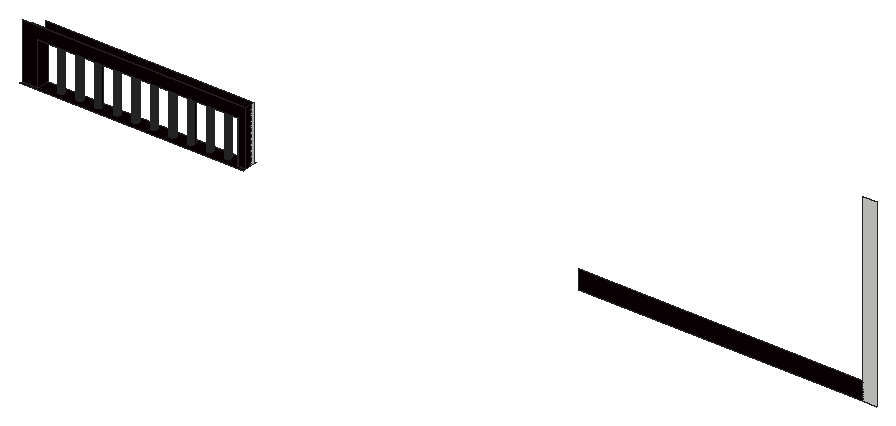
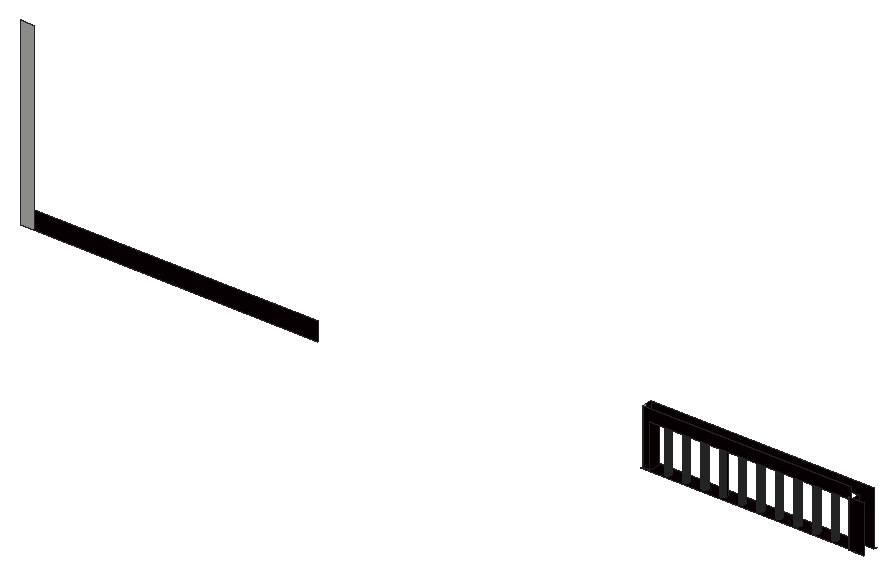
# SketchUp Ruby script. Lengths in inches.
U = 1.inch
M = Sketchup.active_model
def pt(a) = Geom::Point3d.new(a.map { |v| v * U })
def face(e, loops, mat)
  f = e.add_face(loops[0].map { |a| pt(a) })
  loops[1..].each { |l| e.add_face(l.map { |a| pt(a) }).erase! }
  f.material = f.back_material = mat if mat
  f
end
# faces: each face lists its corners as indices into pts; further lists are holes
def faces(e, pts, list, mat = nil) = list.each { |f| face(e, (f[0].is_a?(Array) ? f : [f]).map { |l| l.map { |i| pts[i] } }, mat) }
# xy, xz, yz: faces in a plane at the given z, y or x. An outline is a flat list of corners, or four numbers for a rectangle; further outlines are holes
def ring(l) = l.size == 4 ? [[l[0], l[1]], [l[2], l[1]], [l[2], l[3]], [l[0], l[3]]] : l.each_slice(2).to_a
def flat(e, list, mat, &to3) = list.each { |f| face(e, (f[0].is_a?(Array) ? f : [f]).map { |l| ring(l).map { |u, v| to3.(u, v) } }, mat) }
def xy(e, z, list, mat = nil) = flat(e, list, mat) { |x, y| [x, y, z] }
def xz(e, y, list, mat = nil) = flat(e, list, mat) { |x, z| [x, y, z] }
def yz(e, x, list, mat = nil) = flat(e, list, mat) { |y, z| [x, y, z] }
def lines(e, pts, list) = list.each { |a, b| e.add_line(pt(pts[a]), pt(pts[b])) }
# prism: a flat outline (further loops are holes) pulled along v
def prism(e, loops, v, mat = nil)
  f = face(e, loops, mat); d = Geom::Vector3d.new(v.map { |x| x * U })
  f.pushpull(f.normal.samedirection?(d) ? d.length : -d.length)
end
def box(e, o, s, mat = nil) = prism(e, [[o, [o[0] + s[0], o[1], o[2]], [o[0] + s[0], o[1] + s[1], o[2]], [o[0], o[1] + s[1], o[2]]]], [0, 0, s[2]], mat)
def at(x, y, z, deg = 0) = Geom::Transformation.translation(pt([x, y, z])) * Geom::Transformation.rotation(ORIGIN, Z_AXIS, deg.degrees)
def axes(o, x, y, z) = Geom::Transformation.new([*x, 0, *y, 0, *z, 0, *pt(o).to_a, 1])
def part(name) = M.definitions.add(name)
# library, detail: a bought-in or finely detailed component or shape, given as its bounding box
def library(name, o, s) = part(name).tap { |d| box(d.entities, o, s) }
def detail(e, o, s) = box(e.add_group.entities, o, s)
def put(e, d, t, mat = nil) = e.add_instance(d, t).tap { |i| i.material = mat if mat }
def group(e, t, mat = nil) = e.add_group.tap { |g| g.transformation = t; g.material = mat if mat }.entities
root = M.entities
M.materials.add("[Metal Seamed]").color = [11, 0, 4]
xy(root,288,[[33.7,65.03,33.21,65.13,32.75,65.36,32.38,65.7,32.1,66.12,31.95,66.6,31.92,67.11,32.02,67.6,32.25,68.05,32.59,68.43,33.02,68.71,33.5,68.86,34,68.89,34.5,68.78,34.95,68.55,35.32,68.22,35.6,67.79,35.76,67.3125,35.78,66.81,35.68,66.3125,35.45,65.86,35.11,65.48,34.6875,65.21,34.2,65.05],[45.89,65.03,45.39,65.13,44.94,65.36,44.57,65.7,44.29,66.12,44.13,66.6,44.11,67.11,44.21,67.6,44.44,68.05,44.78,68.43,45.2,68.71,45.68,68.86,46.1875,68.89,46.68,68.78,47.13,68.55,47.51,68.22,47.79,67.79,47.94,67.3125,47.97,66.81,47.86,66.3125,47.64,65.86,47.3,65.48,46.875,65.21,46.39,65.05],[58.07,65.03,57.58,65.13,57.13,65.36,56.75,65.7,56.48,66.12,56.32,66.6,56.29,67.11,56.4,67.6,56.63,68.05,56.97,68.43,57.39,68.71,57.87,68.86,58.375,68.89,58.87,68.78,59.32,68.55,59.7,68.22,59.97,67.79,60.13,67.3125,60.16,66.81,60.05,66.3125,59.82,65.86,59.48,65.48,59.0625,65.21,58.58,65.05],[70.26,65.03,69.77,65.13,69.32,65.36,68.94,65.7,68.66,66.12,68.51,66.6,68.48,67.11,68.59,67.6,68.82,68.05,69.15,68.43,69.58,68.71,70.06,68.86,70.5625,68.89,71.06,68.78,71.51,68.55,71.89,68.22,72.16,67.79,72.32,67.3125,72.34,66.81,72.24,66.3125,72.01,65.86,71.67,65.48,71.25,65.21,70.77,65.05],[82.45,65.03,81.96,65.13,81.5,65.36,81.13,65.7,80.85,66.12,80.7,66.6,80.67,67.11,80.77,67.6,81,68.05,81.34,68.43,81.77,68.71,82.25,68.86,82.75,68.89,83.25,68.78,83.7,68.55,84.07,68.22,84.35,67.79,84.51,67.3125,84.53,66.81,84.43,66.3125,84.2,65.86,83.86,65.48,83.4375,65.21,82.95,65.05],
  [94.64,65.03,94.14,65.13,93.69,65.36,93.32,65.7,93.04,66.12,92.88,66.6,92.86,67.11,92.96,67.6,93.19,68.05,93.53,68.43,93.95,68.71,94.43,68.86,94.9375,68.89,95.43,68.78,95.88,68.55,96.26,68.22,96.54,67.79,96.69,67.3125,96.72,66.81,96.61,66.3125,96.39,65.86,96.05,65.48,95.625,65.21,95.14,65.05],[106.82,65.03,106.33,65.13,105.88,65.36,105.5,65.7,105.23,66.12,105.07,66.6,105.04,67.11,105.15,67.6,105.38,68.05,105.72,68.43,106.14,68.71,106.62,68.86,107.125,68.89,107.62,68.78,108.07,68.55,108.45,68.22,108.72,67.79,108.88,67.3125,108.91,66.81,108.8,66.3125,108.57,65.86,108.23,65.48,107.8125,65.21,107.33,65.05],[119.01,65.03,118.52,65.13,118.07,65.36,117.69,65.7,117.41,66.12,117.26,66.6,117.23,67.11,117.34,67.6,117.57,68.05,117.9,68.43,118.33,68.71,118.81,68.86,119.3125,68.89,119.81,68.78,120.26,68.55,120.64,68.22,120.91,67.79,121.07,67.3125,121.09,66.81,120.99,66.3125,120.76,65.86,120.42,65.48,120,65.21,119.52,65.05],[131.2,65.03,130.71,65.13,130.25,65.36,129.88,65.7,129.6,66.12,129.45,66.6,129.42,67.11,129.52,67.6,129.75,68.05,130.09,68.43,130.52,68.71,131,68.86,131.5,68.89,132,68.78,132.45,68.55,132.82,68.22,133.1,67.79,133.26,67.3125,133.28,66.81,133.18,66.3125,132.95,65.86,132.61,65.48,132.1875,65.21,131.7,65.05],[143.07,65.03,142.58,65.13,142.13,65.36,141.75,65.7,141.48,66.12,141.32,66.6,141.29,67.11,141.4,67.6,141.63,68.05,141.97,68.43,142.39,68.71,142.87,68.86,143.375,68.89,143.87,68.78,144.32,68.55,144.7,68.22,144.97,67.79,145.13,67.3125,145.16,66.81,145.05,66.3125,144.82,65.86,144.48,65.48,144.0625,65.21,143.58,65.05],
  [16.88,66.64,17.49,66.68,18.05,66.88,18.55,67.22,18.95,67.68,19.21,68.22,19.32,68.82,19.28,69.42,19.08,69.99,18.74,70.49,18.28,70.88,17.77,71.13,16.3,71.13,15.97,71.01,15.47,70.67,15.08,70.21,14.82,69.67,14.7,69.08,14.75,68.48,14.95,67.91,15.29,67.41,15.75,67.01,16.29,66.75],[16.3,71.13,17.77,71.13,17.74,71.14,17.14,71.26,16.54,71.21]])
xy(root,288,[[[11.6875,61.03,158,61.03,158,62.76,153.04,62.76,153.04,69.57,158,69.57,158,70.73,21.75,70.73,21.75,62.76,11.6875,62.76],[33.7,65.03,33.21,65.13,32.75,65.36,32.38,65.7,32.1,66.12,31.95,66.6,31.92,67.11,32.02,67.6,32.25,68.05,32.59,68.43,33.02,68.71,33.5,68.86,34,68.89,34.5,68.78,34.95,68.55,35.32,68.22,35.6,67.79,35.76,67.3125,35.78,66.81,35.68,66.3125,35.45,65.86,35.11,65.48,34.6875,65.21,34.2,65.05],[45.89,65.03,45.39,65.13,44.94,65.36,44.57,65.7,44.29,66.12,44.13,66.6,44.11,67.11,44.21,67.6,44.44,68.05,44.78,68.43,45.2,68.71,45.68,68.86,46.1875,68.89,46.68,68.78,47.13,68.55,47.51,68.22,47.79,67.79,47.94,67.3125,47.97,66.81,47.86,66.3125,47.64,65.86,47.3,65.48,46.875,65.21,46.39,65.05],[58.07,65.03,57.58,65.13,57.13,65.36,56.75,65.7,56.48,66.12,56.32,66.6,56.29,67.11,56.4,67.6,56.63,68.05,56.97,68.43,57.39,68.71,57.87,68.86,58.375,68.89,58.87,68.78,59.32,68.55,59.7,68.22,59.97,67.79,60.13,67.3125,60.16,66.81,60.05,66.3125,59.82,65.86,59.48,65.48,59.0625,65.21,58.58,65.05],[70.26,65.03,69.77,65.13,69.32,65.36,68.94,65.7,68.66,66.12,68.51,66.6,68.48,67.11,68.59,67.6,68.82,68.05,69.15,68.43,69.58,68.71,70.06,68.86,70.5625,68.89,71.06,68.78,71.51,68.55,71.89,68.22,72.16,67.79,72.32,67.3125,72.34,66.81,72.24,66.3125,72.01,65.86,71.67,65.48,71.25,65.21,70.77,65.05],[82.45,65.03,81.96,65.13,81.5,65.36,81.13,65.7,80.85,66.12,80.7,66.6,80.67,67.11,80.77,67.6,81,68.05,81.34,68.43,81.77,68.71,82.25,68.86,82.75,68.89,83.25,68.78,83.7,68.55,84.07,68.22,84.35,67.79,84.51,67.3125,84.53,66.81,84.43,66.3125,84.2,65.86,83.86,65.48,83.4375,65.21,82.95,65.05],[94.64,65.03,94.14,65.13,93.69,65.36,93.32,65.7,93.04,66.12,92.88,66.6,92.86,67.11,92.96,67.6,93.19,68.05,93.53,68.43,93.95,68.71,94.43,68.86,94.9375,68.89,95.43,68.78,95.88,68.55,96.26,68.22,96.54,67.79,96.69,67.3125,96.72,66.81,96.61,66.3125,96.39,65.86,96.05,65.48,95.625,65.21,95.14,65.05],[106.82,65.03,106.33,65.13,105.88,65.36,105.5,65.7,105.23,66.12,105.07,66.6,105.04,67.11,105.15,67.6,105.38,68.05,105.72,68.43,106.14,68.71,106.62,68.86,107.125,68.89,107.62,68.78,108.07,68.55,108.45,68.22,108.72,67.79,108.88,67.3125,108.91,66.81,108.8,66.3125,108.57,65.86,108.23,65.48,107.8125,65.21,107.33,65.05],[119.01,65.03,118.52,65.13,118.07,65.36,117.69,65.7,117.41,66.12,117.26,66.6,117.23,67.11,117.34,67.6,117.57,68.05,117.9,68.43,118.33,68.71,118.81,68.86,119.3125,68.89,119.81,68.78,120.26,68.55,120.64,68.22,120.91,67.79,121.07,67.3125,121.09,66.81,120.99,66.3125,120.76,65.86,120.42,65.48,120,65.21,119.52,65.05],[131.2,65.03,130.71,65.13,130.25,65.36,129.88,65.7,129.6,66.12,129.45,66.6,129.42,67.11,129.52,67.6,129.75,68.05,130.09,68.43,130.52,68.71,131,68.86,131.5,68.89,132,68.78,132.45,68.55,132.82,68.22,133.1,67.79,133.26,67.3125,133.28,66.81,133.18,66.3125,132.95,65.86,132.61,65.48,132.1875,65.21,131.7,65.05],[143.07,65.03,142.58,65.13,142.13,65.36,141.75,65.7,141.48,66.12,141.32,66.6,141.29,67.11,141.4,67.6,141.63,68.05,141.97,68.43,142.39,68.71,142.87,68.86,143.375,68.89,143.87,68.78,144.32,68.55,144.7,68.22,144.97,67.79,145.13,67.3125,145.16,66.81,145.05,66.3125,144.82,65.86,144.48,65.48,144.0625,65.21,143.58,65.05]]],"[Metal Seamed]")
xz(root,62.76,[[11.6875,288,21.75,288,21.75,316.34,153.04,316.34,153.04,288,158,288,158,324,11.6875,324]],"[Metal Seamed]")
xz(root,69.57,[[153.04,288,153.04,316.34,21.75,316.34,21.75,324,158,324,158,288]],"[Metal Seamed]")
xz(root,70.97,[[555.7,288,564.5,408]])
xz(root,70.97,[[369.3125,288,555.7,300]],"[Metal Seamed]")
xz(root,71.13,[[11.6875,288,21.75,318.96]],"[Metal Seamed]")
yz(root,21.75,[[62.76,288,71.13,288,71.13,317.84,69.57,317.84,69.57,316.34,62.76,316.34]],"[Metal Seamed]")
yz(root,153.04,[[62.76,288,69.57,316.34]],"[Metal Seamed]")
yz(root,158,[[67.28,288,69.57,324]])
yz(root,158,[[62.76,288,67.28,324]],"[Metal Seamed]")
p = [[33.21,65.13,288],[33.7,65.03,288],[33.7,65.03,316.34],[33.21,65.13,316.34],[34.2,65.05,288],[34.2,65.05,316.34],
  [45.39,65.13,288],[45.89,65.03,288],[45.89,65.03,316.6875],[45.39,65.13,316.6875],[46.39,65.05,288],[46.39,65.05,316.6875],
  [57.58,65.13,288],[58.07,65.03,288],[58.07,65.03,317.375],[57.58,65.13,317.375],[58.58,65.05,288],[58.58,65.05,317.375],
  [69.77,65.13,288],[70.26,65.03,288],[70.26,65.03,317.6875],[69.77,65.13,317.6875],[70.77,65.05,288],[70.77,65.05,317.6875],
  [81.96,65.13,288],[82.45,65.03,288],[82.45,65.03,317.4375],[81.96,65.13,317.4375],[82.95,65.05,288],[82.95,65.05,317.4375],
  [94.14,65.13,288],[94.64,65.03,288],[94.64,65.03,319.8125],[94.14,65.13,319.8125],[95.14,65.05,288],[95.14,65.05,319.8125],
  [106.33,65.13,288],[106.82,65.03,288],[106.82,65.03,319.125],[106.33,65.13,319.125],[107.33,65.05,288],[107.33,65.05,319.125],
  [118.52,65.13,288],[119.01,65.03,288],[119.01,65.03,318.9375],[118.52,65.13,318.9375],[119.52,65.05,288],[119.52,65.05,318.9375],
  [130.71,65.13,288],[131.2,65.03,288],[131.2,65.03,318.625],[130.71,65.13,318.625],[131.7,65.05,288],[131.7,65.05,318.625],
  [142.58,65.13,288],[143.07,65.03,288],[143.07,65.03,317.5],[142.58,65.13,317.5],[143.58,65.05,288],[143.58,65.05,317.5],
  [32.75,65.36,288],[32.75,65.36,316.34],[34.6875,65.21,288],[34.6875,65.21,316.34],[44.94,65.36,288],[44.94,65.36,316.6875],
  [46.875,65.21,288],[46.875,65.21,316.6875],[57.13,65.36,288],[57.13,65.36,317.375],[59.0625,65.21,288],[59.0625,65.21,317.375],
  [69.32,65.36,288],[69.32,65.36,317.6875],[71.25,65.21,288],[71.25,65.21,317.6875],[81.5,65.36,288],[81.5,65.36,317.4375],
  [83.4375,65.21,288],[83.4375,65.21,317.4375],[93.69,65.36,288],[93.69,65.36,319.8125],[95.625,65.21,288],[95.625,65.21,319.8125],
  [105.88,65.36,288],[105.88,65.36,319.125],[107.8125,65.21,288],[107.8125,65.21,319.125],[118.07,65.36,288],[118.07,65.36,318.9375],
  [120,65.21,288],[120,65.21,318.9375],[130.25,65.36,288],[130.25,65.36,318.625],[132.1875,65.21,288],[132.1875,65.21,318.625],
  [142.13,65.36,288],[142.13,65.36,317.5],[144.0625,65.21,288],[144.0625,65.21,317.5],[35.11,65.48,288],[35.11,65.48,316.34],
  [47.3,65.48,288],[47.3,65.48,316.6875],[59.48,65.48,288],[59.48,65.48,317.375],[71.67,65.48,288],[71.67,65.48,317.6875],
  [83.86,65.48,288],[83.86,65.48,317.4375],[96.05,65.48,288],[96.05,65.48,319.8125],[108.23,65.48,288],[108.23,65.48,319.125],
  [120.42,65.48,288],[120.42,65.48,318.9375],[132.61,65.48,288],[132.61,65.48,318.625],[144.48,65.48,288],[144.48,65.48,317.5],
  [32.38,65.7,288],[32.38,65.7,316.34],[44.57,65.7,288],[44.57,65.7,316.6875],[56.75,65.7,288],[56.75,65.7,317.375],
  [68.94,65.7,288],[68.94,65.7,317.6875],[81.13,65.7,288],[81.13,65.7,317.4375],[93.32,65.7,288],[93.32,65.7,319.8125],
  [105.5,65.7,288],[105.5,65.7,319.125],[117.69,65.7,288],[117.69,65.7,318.9375],[129.88,65.7,288],[129.88,65.7,318.625],
  [141.75,65.7,288],[141.75,65.7,317.5],[35.45,65.86,288],[35.45,65.86,316.34],[47.64,65.86,288],[47.64,65.86,316.6875],
  [59.82,65.86,288],[59.82,65.86,317.375],[72.01,65.86,288],[72.01,65.86,317.6875],[84.2,65.86,288],[84.2,65.86,317.4375],
  [96.39,65.86,288],[96.39,65.86,319.8125],[108.57,65.86,288],[108.57,65.86,319.125],[120.76,65.86,288],[120.76,65.86,318.9375],
  [132.95,65.86,288],[132.95,65.86,318.625],[144.82,65.86,288],[144.82,65.86,317.5],[32.1,66.12,288],[32.1,66.12,316.34],
  [44.29,66.12,288],[44.29,66.12,316.6875],[56.48,66.12,288],[56.48,66.12,317.375],[68.66,66.12,288],[68.66,66.12,317.6875],
  [80.85,66.12,288],[80.85,66.12,317.4375],[93.04,66.12,288],[93.04,66.12,319.8125],[105.23,66.12,288],[105.23,66.12,319.125],
  [117.41,66.12,288],[117.41,66.12,318.9375],[129.6,66.12,288],[129.6,66.12,318.625],[141.48,66.12,288],[141.48,66.12,317.5],
  [35.68,66.3125,288],[35.68,66.3125,316.34],[47.86,66.3125,288],[47.86,66.3125,316.6875],[60.05,66.3125,288],[60.05,66.3125,317.375],
  [72.24,66.3125,288],[72.24,66.3125,317.6875],[84.43,66.3125,288],[84.43,66.3125,317.4375],[96.61,66.3125,288],[96.61,66.3125,319.8125],
  [108.8,66.3125,288],[108.8,66.3125,319.125],[120.99,66.3125,288],[120.99,66.3125,318.9375],[133.18,66.3125,288],[133.18,66.3125,318.625],
  [145.05,66.3125,288],[145.05,66.3125,317.5],[31.95,66.6,288],[31.95,66.6,316.34],[44.13,66.6,288],[44.13,66.6,316.6875],
  [56.32,66.6,288],[56.32,66.6,317.375],[68.51,66.6,288],[68.51,66.6,317.6875],[80.7,66.6,288],[80.7,66.6,317.4375],
  [92.88,66.6,288],[92.88,66.6,319.8125],[105.07,66.6,288],[105.07,66.6,319.125],[117.26,66.6,288],[117.26,66.6,318.9375],
  [129.45,66.6,288],[129.45,66.6,318.625],[141.32,66.6,288],[141.32,66.6,317.5],[35.78,66.81,288],[35.78,66.81,316.34],
  [47.97,66.81,288],[47.97,66.81,316.6875],[60.16,66.81,288],[60.16,66.81,317.375],[72.34,66.81,288],[72.34,66.81,317.6875],
  [84.53,66.81,288],[84.53,66.81,317.4375],[96.72,66.81,288],[96.72,66.81,319.8125],[108.91,66.81,288],[108.91,66.81,319.125],
  [121.09,66.81,288],[121.09,66.81,318.9375],[133.28,66.81,288],[133.28,66.81,318.625],[145.16,66.81,288],[145.16,66.81,317.5],
  [31.92,67.11,288],[31.92,67.11,316.34],[44.11,67.11,288],[44.11,67.11,316.6875],[56.29,67.11,288],[56.29,67.11,317.375],
  [68.48,67.11,288],[68.48,67.11,317.6875],[80.67,67.11,288],[80.67,67.11,317.4375],[92.86,67.11,288],[92.86,67.11,319.8125],
  [105.04,67.11,288],[105.04,67.11,319.125],[117.23,67.11,288],[117.23,67.11,318.9375],[129.42,67.11,288],[129.42,67.11,318.625],
  [141.29,67.11,288],[141.29,67.11,317.5],[35.76,67.3125,288],[35.76,67.3125,316.34],[47.94,67.3125,288],[47.94,67.3125,316.6875],
  [60.13,67.3125,288],[60.13,67.3125,317.375],[72.32,67.3125,288],[72.32,67.3125,317.6875],[84.51,67.3125,288],[84.51,67.3125,317.4375],
  [96.69,67.3125,288],[96.69,67.3125,319.8125],[108.88,67.3125,288],[108.88,67.3125,319.125],[121.07,67.3125,288],[121.07,67.3125,318.9375],
  [133.26,67.3125,288],[133.26,67.3125,318.625],[145.13,67.3125,288],[145.13,67.3125,317.5],[32.02,67.6,288],[32.02,67.6,316.34],
  [44.21,67.6,288],[44.21,67.6,316.6875],[56.4,67.6,288],[56.4,67.6,317.375],[68.59,67.6,288],[68.59,67.6,317.6875],
  [80.77,67.6,288],[80.77,67.6,317.4375],[92.96,67.6,288],[92.96,67.6,319.8125],[105.15,67.6,288],[105.15,67.6,319.125],
  [117.34,67.6,288],[117.34,67.6,318.9375],[129.52,67.6,288],[129.52,67.6,318.625],[141.4,67.6,288],[141.4,67.6,317.5],
  [35.6,67.79,288],[35.6,67.79,316.34],[47.79,67.79,288],[47.79,67.79,316.6875],[59.97,67.79,288],[59.97,67.79,317.375],
  [72.16,67.79,288],[72.16,67.79,317.6875],[84.35,67.79,288],[84.35,67.79,317.4375],[96.54,67.79,288],[96.54,67.79,319.8125],
  [108.72,67.79,288],[108.72,67.79,319.125],[120.91,67.79,288],[120.91,67.79,318.9375],[133.1,67.79,288],[133.1,67.79,318.625],
  [144.97,67.79,288],[144.97,67.79,317.5],[32.25,68.05,288],[32.25,68.05,316.34],[44.44,68.05,288],[44.44,68.05,316.6875],
  [56.63,68.05,288],[56.63,68.05,317.375],[68.82,68.05,288],[68.82,68.05,317.6875],[81,68.05,288],[81,68.05,317.4375],
  [93.19,68.05,288],[93.19,68.05,319.8125],[105.38,68.05,288],[105.38,68.05,319.125],[117.57,68.05,288],[117.57,68.05,318.9375],
  [129.75,68.05,288],[129.75,68.05,318.625],[141.63,68.05,288],[141.63,68.05,317.5],[35.32,68.22,288],[35.32,68.22,316.34],
  [47.51,68.22,288],[47.51,68.22,316.6875],[59.7,68.22,288],[59.7,68.22,317.375],[71.89,68.22,288],[71.89,68.22,317.6875],
  [84.07,68.22,288],[84.07,68.22,317.4375],[96.26,68.22,288],[96.26,68.22,319.8125],[108.45,68.22,288],[108.45,68.22,319.125],
  [120.64,68.22,288],[120.64,68.22,318.9375],[132.82,68.22,288],[132.82,68.22,318.625],[144.7,68.22,288],[144.7,68.22,317.5],
  [32.59,68.43,288],[32.59,68.43,316.34],[44.78,68.43,288],[44.78,68.43,316.6875],[56.97,68.43,288],[56.97,68.43,317.375],
  [69.15,68.43,288],[69.15,68.43,317.6875],[81.34,68.43,288],[81.34,68.43,317.4375],[93.53,68.43,288],[93.53,68.43,319.8125],
  [105.72,68.43,288],[105.72,68.43,319.125],[117.9,68.43,288],[117.9,68.43,318.9375],[130.09,68.43,288],[130.09,68.43,318.625],
  [141.97,68.43,288],[141.97,68.43,317.5],[34.95,68.55,288],[34.95,68.55,316.34],[47.13,68.55,288],[47.13,68.55,316.6875],
  [59.32,68.55,288],[59.32,68.55,317.375],[71.51,68.55,288],[71.51,68.55,317.6875],[83.7,68.55,288],[83.7,68.55,317.4375],
  [95.88,68.55,288],[95.88,68.55,319.8125],[108.07,68.55,288],[108.07,68.55,319.125],[120.26,68.55,288],[120.26,68.55,318.9375],
  [132.45,68.55,288],[132.45,68.55,318.625],[144.32,68.55,288],[144.32,68.55,317.5],[33.02,68.71,288],[33.02,68.71,316.34],
  [45.2,68.71,288],[45.2,68.71,316.6875],[57.39,68.71,288],[57.39,68.71,317.375],[69.58,68.71,288],[69.58,68.71,317.6875],
  [81.77,68.71,288],[81.77,68.71,317.4375],[93.95,68.71,288],[93.95,68.71,319.8125],[106.14,68.71,288],[106.14,68.71,319.125],
  [118.33,68.71,288],[118.33,68.71,318.9375],[130.52,68.71,288],[130.52,68.71,318.625],[142.39,68.71,288],[142.39,68.71,317.5],
  [34.5,68.78,288],[34.5,68.78,316.34],[46.68,68.78,288],[46.68,68.78,316.6875],[58.87,68.78,288],[58.87,68.78,317.375],
  [71.06,68.78,288],[71.06,68.78,317.6875],[83.25,68.78,288],[83.25,68.78,317.4375],[95.43,68.78,288],[95.43,68.78,319.8125],
  [107.62,68.78,288],[107.62,68.78,319.125],[119.81,68.78,288],[119.81,68.78,318.9375],[132,68.78,288],[132,68.78,318.625],
  [143.87,68.78,288],[143.87,68.78,317.5],[33.5,68.86,288],[33.5,68.86,316.34],[45.68,68.86,288],[45.68,68.86,316.6875],
  [57.87,68.86,288],[57.87,68.86,317.375],[70.06,68.86,288],[70.06,68.86,317.6875],[82.25,68.86,288],[82.25,68.86,317.4375],
  [94.43,68.86,288],[94.43,68.86,319.8125],[106.62,68.86,288],[106.62,68.86,319.125],[118.81,68.86,288],[118.81,68.86,318.9375],
  [131,68.86,288],[131,68.86,318.625],[142.87,68.86,288],[142.87,68.86,317.5],[34,68.89,288],[34,68.89,316.34],
  [46.1875,68.89,288],[46.1875,68.89,316.6875],[58.375,68.89,288],[58.375,68.89,317.375],[70.5625,68.89,288],[70.5625,68.89,317.6875],
  [82.75,68.89,288],[82.75,68.89,317.4375],[94.9375,68.89,288],[94.9375,68.89,319.8125],[107.125,68.89,288],[107.125,68.89,319.125],
  [119.3125,68.89,288],[119.3125,68.89,318.9375],[131.5,68.89,288],[131.5,68.89,318.625],[143.375,68.89,288],[143.375,68.89,317.5]]
faces(root,p,[[0,1,2,3],[1,4,5,2],[6,7,8,9],[7,10,11,8],[12,13,14,15],[13,16,17,14],[18,19,20,21],[19,22,23,20],
  [24,25,26,27],[25,28,29,26],[30,31,32,33],[31,34,35,32],[36,37,38,39],[37,40,41,38],[42,43,44,45],[43,46,47,44],
  [48,49,50,51],[49,52,53,50],[54,55,56,57],[55,58,59,56],[60,0,3,61],[4,62,63,5],[64,6,9,65],[10,66,67,11],
  [68,12,15,69],[16,70,71,17],[72,18,21,73],[22,74,75,23],[76,24,27,77],[28,78,79,29],[80,30,33,81],[34,82,83,35],
  [84,36,39,85],[40,86,87,41],[88,42,45,89],[46,90,91,47],[92,48,51,93],[52,94,95,53],[96,54,57,97],[58,98,99,59],
  [62,100,101,63],[66,102,103,67],[70,104,105,71],[74,106,107,75],[78,108,109,79],[82,110,111,83],[86,112,113,87],[90,114,115,91],
  [94,116,117,95],[98,118,119,99],[120,60,61,121],[122,64,65,123],[124,68,69,125],[126,72,73,127],[128,76,77,129],[130,80,81,131],
  [132,84,85,133],[134,88,89,135],[136,92,93,137],[138,96,97,139],[100,140,141,101],[102,142,143,103],[104,144,145,105],[106,146,147,107],
  [108,148,149,109],[110,150,151,111],[112,152,153,113],[114,154,155,115],[116,156,157,117],[118,158,159,119],[160,120,121,161],[162,122,123,163],
  [164,124,125,165],[166,126,127,167],[168,128,129,169],[170,130,131,171],[172,132,133,173],[174,134,135,175],[176,136,137,177],[178,138,139,179],
  [140,180,181,141],[142,182,183,143],[144,184,185,145],[146,186,187,147],[148,188,189,149],[150,190,191,151],[152,192,193,153],[154,194,195,155],
  [156,196,197,157],[158,198,199,159],[200,160,161,201],[202,162,163,203],[204,164,165,205],[206,166,167,207],[208,168,169,209],[210,170,171,211],
  [212,172,173,213],[214,174,175,215],[216,176,177,217],[218,178,179,219],[180,220,221,181],[182,222,223,183],[184,224,225,185],[186,226,227,187],
  [188,228,229,189],[190,230,231,191],[192,232,233,193],[194,234,235,195],[196,236,237,197],[198,238,239,199],[240,200,201,241],[242,202,203,243],
  [244,204,205,245],[246,206,207,247],[248,208,209,249],[250,210,211,251],[252,212,213,253],[254,214,215,255],[256,216,217,257],[258,218,219,259],
  [220,260,261,221],[222,262,263,223],[224,264,265,225],[226,266,267,227],[228,268,269,229],[230,270,271,231],[232,272,273,233],[234,274,275,235],
  [236,276,277,237],[238,278,279,239],[280,240,241,281],[282,242,243,283],[284,244,245,285],[286,246,247,287],[288,248,249,289],[290,250,251,291],
  [292,252,253,293],[294,254,255,295],[296,256,257,297],[298,258,259,299],[260,300,301,261],[262,302,303,263],[264,304,305,265],[266,306,307,267],
  [268,308,309,269],[270,310,311,271],[272,312,313,273],[274,314,315,275],[276,316,317,277],[278,318,319,279],[320,280,281,321],[322,282,283,323],
  [324,284,285,325],[326,286,287,327],[328,288,289,329],[330,290,291,331],[332,292,293,333],[334,294,295,335],[336,296,297,337],[338,298,299,339],
  [300,340,341,301],[302,342,343,303],[304,344,345,305],[306,346,347,307],[308,348,349,309],[310,350,351,311],[312,352,353,313],[314,354,355,315],
  [316,356,357,317],[318,358,359,319],[360,320,321,361],[362,322,323,363],[364,324,325,365],[366,326,327,367],[368,328,329,369],[370,330,331,371],
  [372,332,333,373],[374,334,335,375],[376,336,337,377],[378,338,339,379],[340,380,381,341],[342,382,383,343],[344,384,385,345],[346,386,387,347],
  [348,388,389,349],[350,390,391,351],[352,392,393,353],[354,394,395,355],[356,396,397,357],[358,398,399,359],[400,360,361,401],[402,362,363,403],
  [404,364,365,405],[406,366,367,407],[408,368,369,409],[410,370,371,411],[412,372,373,413],[414,374,375,415],[416,376,377,417],[418,378,379,419],
  [380,420,421,381],[382,422,423,383],[384,424,425,385],[386,426,427,387],[388,428,429,389],[390,430,431,391],[392,432,433,393],[394,434,435,395],
  [396,436,437,397],[398,438,439,399],[440,400,401,441],[442,402,403,443],[444,404,405,445],[446,406,407,447],[448,408,409,449],[450,410,411,451],
  [452,412,413,453],[454,414,415,455],[456,416,417,457],[458,418,419,459],[420,460,461,421],[422,462,463,423],[424,464,465,425],[426,466,467,427],
  [428,468,469,429],[430,470,471,431],[432,472,473,433],[434,474,475,435],[436,476,477,437],[438,478,479,439],[460,440,441,461],[462,442,443,463],
  [464,444,445,465],[466,446,447,467],[468,448,449,469],[470,450,451,471],[472,452,453,473],[474,454,455,475],[476,456,457,477],[478,458,459,479]],"[Metal Seamed]")
